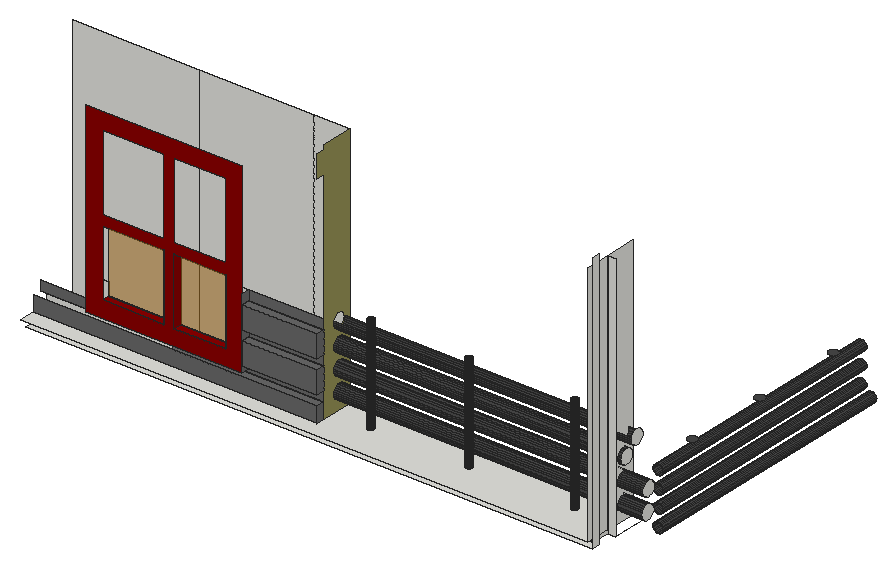
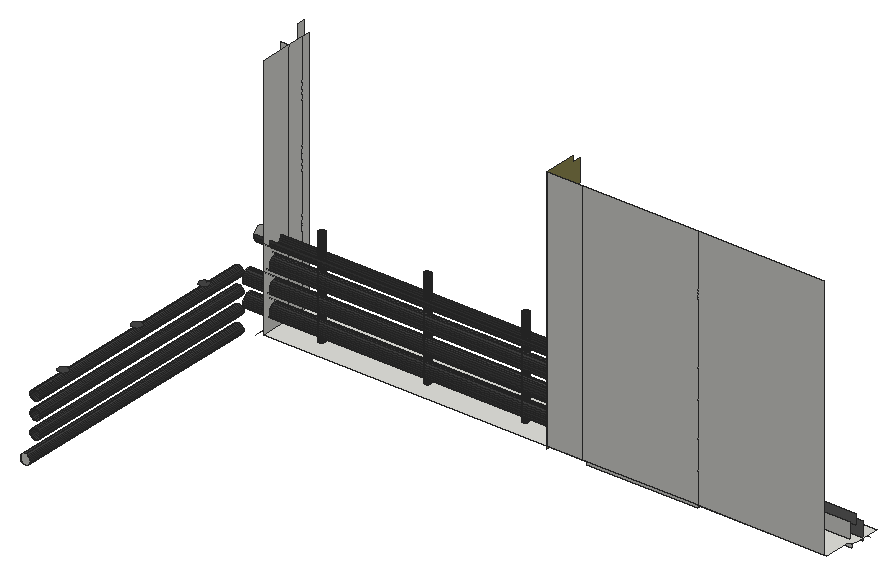
# SketchUp Ruby script. Lengths in inches.
U = 1.inch
M = Sketchup.active_model
def pt(a) = Geom::Point3d.new(a.map { |v| v * U })
def face(e, loops, mat)
  f = e.add_face(loops[0].map { |a| pt(a) })
  loops[1..].each { |l| e.add_face(l.map { |a| pt(a) }).erase! }
  f.material = f.back_material = mat if mat
  f
end
# faces: each face lists its corners as indices into pts; further lists are holes
def faces(e, pts, list, mat = nil) = list.each { |f| face(e, (f[0].is_a?(Array) ? f : [f]).map { |l| l.map { |i| pts[i] } }, mat) }
# xy, xz, yz: faces in a plane at the given z, y or x. An outline is a flat list of corners, or four numbers for a rectangle; further outlines are holes
def ring(l) = l.size == 4 ? [[l[0], l[1]], [l[2], l[1]], [l[2], l[3]], [l[0], l[3]]] : l.each_slice(2).to_a
def flat(e, list, mat, &to3) = list.each { |f| face(e, (f[0].is_a?(Array) ? f : [f]).map { |l| ring(l).map { |u, v| to3.(u, v) } }, mat) }
def xy(e, z, list, mat = nil) = flat(e, list, mat) { |x, y| [x, y, z] }
def xz(e, y, list, mat = nil) = flat(e, list, mat) { |x, z| [x, y, z] }
def yz(e, x, list, mat = nil) = flat(e, list, mat) { |y, z| [x, y, z] }
def lines(e, pts, list) = list.each { |a, b| e.add_line(pt(pts[a]), pt(pts[b])) }
# prism: a flat outline (further loops are holes) pulled along v
def prism(e, loops, v, mat = nil)
  f = face(e, loops, mat); d = Geom::Vector3d.new(v.map { |x| x * U })
  f.pushpull(f.normal.samedirection?(d) ? d.length : -d.length)
end
def box(e, o, s, mat = nil) = prism(e, [[o, [o[0] + s[0], o[1], o[2]], [o[0] + s[0], o[1] + s[1], o[2]], [o[0], o[1] + s[1], o[2]]]], [0, 0, s[2]], mat)
def at(x, y, z, deg = 0) = Geom::Transformation.translation(pt([x, y, z])) * Geom::Transformation.rotation(ORIGIN, Z_AXIS, deg.degrees)
def axes(o, x, y, z) = Geom::Transformation.new([*x, 0, *y, 0, *z, 0, *pt(o).to_a, 1])
def part(name) = M.definitions.add(name)
# library, detail: a bought-in or finely detailed component or shape, given as its bounding box
def library(name, o, s) = part(name).tap { |d| box(d.entities, o, s) }
def detail(e, o, s) = box(e.add_group.entities, o, s)
def put(e, d, t, mat = nil) = e.add_instance(d, t).tap { |i| i.material = mat if mat }
def group(e, t, mat = nil) = e.add_group.tap { |g| g.transformation = t; g.material = mat if mat }.entities
root = M.entities
M.materials.add("[0021_DarkRed]").color = [139, 0, 0]
M.materials.add("[0057_DarkKhaki]").color = [150, 145, 85]
M.materials.add("[0134_DimGray]").color = [105, 105, 105]
M.materials.add("[0137_Black]").color = [71, 71, 71]
M.materials.add("[Translucent Glass Gray]").color = [191, 123, 24]
M.materials["[Translucent Glass Gray]"].alpha = 0.5
xy(root,135.48,[[286.64,1.0625,497.29,4.0625]])
xy(root,135.98,[[286.99,7.0625,334.1,10.0625],[334.1,7.0625,375.29,10.0625],[375.29,7.0625,390.0625,10.0625],[334.1,10.0625,375.29,22.0625]])
xy(root,137.03,[[[284.41,1.0625,495.71,1.0625,495.71,22.0625,286.17,22.0625,286.17,12.1875,284.66,12.1875,284.66,10.0625,284.41,10.0625],[480.14,13.19,479.85,13.23,479.58,13.34,479.35,13.52,479.17,13.76,479.05,14.03,479.02,14.32,479.05,14.61,479.17,14.88,479.35,15.11,479.58,15.29,479.85,15.41,480.14,15.44,480.43,15.41,480.7,15.29,480.9375,15.11,481.12,14.88,481.23,14.61,481.27,14.32,481.23,14.03,481.12,13.76,480.9375,13.52,480.7,13.34,480.43,13.23],[440.77,13.19,440.47,13.23,440.2,13.34,439.97,13.52,439.79,13.76,439.68,14.03,439.64,14.32,439.68,14.61,439.79,14.88,439.97,15.11,440.2,15.29,440.47,15.41,440.77,15.44,441.06,15.41,441.33,15.29,441.5625,15.11,441.74,14.88,441.85,14.61,441.89,14.32,441.85,14.03,441.74,13.76,441.5625,13.52,441.33,13.34,441.06,13.23],[404.27,13.19,403.97,13.23,403.7,13.34,403.47,13.52,403.29,13.76,403.18,14.03,403.14,14.32,403.18,14.61,403.29,14.88,403.47,15.11,403.7,15.29,403.97,15.41,404.27,15.44,404.56,15.41,404.83,15.29,405.0625,15.11,405.24,14.88,405.35,14.61,405.39,14.32,405.35,14.03,405.24,13.76,405.0625,13.52,404.83,13.34,404.56,13.23]]])
xy(root,142.6875,[[335.53,7.0625,390.0625,10.0625]],"[0134_DimGray]")
xy(root,143.85,[[304.13,7.0625,362.13,10.0625]])
xy(root,146.27,[[362.13,7.0625,390.0625,10.0625]],"[0134_DimGray]")
xy(root,149.85,[[310.13,7.0625,333.13,10.0625],[336.9,7.0625,356.13,10.0625]],"[0021_DarkRed]")
xy(root,154.6875,[[362.13,7.0625,390.0625,10.0625]],"[0134_DimGray]")
xy(root,158.25,[[504.72,36.55,505.18,36.6,505.6,36.78,505.96,37.06,506.24,37.42,506.41,37.84,506.47,38.3,506.41,38.75,506.24,39.17,505.96,39.53,505.6,39.8125,505.18,39.99,504.72,40.05,504.27,39.99,503.85,39.8125,503.49,39.53,503.21,39.17,503.03,38.75,502.97,38.3,503.03,37.84,503.21,37.42,503.49,37.06,503.85,36.78,504.27,36.6],[504.72,67.92,505.18,67.98,505.6,68.15,505.96,68.43,506.24,68.8,506.41,69.22,506.47,69.67,506.41,70.125,506.24,70.55,505.96,70.91,505.6,71.1875,505.18,71.36,504.72,71.42,504.27,71.36,503.85,71.1875,503.49,70.91,503.21,70.55,503.03,70.125,502.97,69.67,503.03,69.22,503.21,68.8,503.49,68.43,503.85,68.15,504.27,67.98],[504.72,102.17,505.18,102.23,505.6,102.4,505.96,102.68,506.24,103.05,506.41,103.47,506.47,103.92,506.41,104.375,506.24,104.8,505.96,105.16,505.6,105.4375,505.18,105.61,504.72,105.67,504.27,105.61,503.85,105.4375,503.49,105.16,503.21,104.8,503.03,104.375,502.97,103.92,503.03,103.47,503.21,103.05,503.49,102.68,503.85,102.4,504.27,102.23]],"[0137_Black]")
xy(root,158.27,[[362.13,7.0625,390.0625,10.0625]],"[0134_DimGray]")
xy(root,166.6875,[[362.13,7.0625,390.0625,10.0625]],"[0134_DimGray]")
xz(root,7.0625,[[[304.13,143.85,362.13,212.79],[310.13,178.32,333.13,206.79],[310.13,149.85,333.13,174.59],[336.9,178.32,356.13,206.79],[336.9,149.85,356.13,174.59]]],"[0021_DarkRed]")
xz(root,7.0625,[[284.66,135.98,390.0625,142.6875],[362.13,146.27,390.0625,154.6875],[362.13,158.27,390.0625,166.6875]],"[0134_DimGray]")
xz(root,10.0625,[[286.17,134.27,390.0625,135.98],[286.99,135.98,390.0625,142.6875],[495.71,135.98,498.65,228.47],[304.13,143.85,362.13,146.27],[304.13,146.27,362.13,146.27,362.13,154.6875,356.13,154.6875,356.13,149.85,336.9,149.85,336.9,154.6875,333.13,154.6875,333.13,149.85,310.13,149.85,310.13,154.6875,304.13,154.6875],
  [362.13,146.27,390.0625,154.6875],[333.13,154.6875,336.9,158.27],[356.13,154.6875,362.13,158.27],[333.13,158.27,336.9,166.6875],[356.13,158.27,362.13,166.6875],
  [362.13,158.27,390.0625,166.6875],[333.13,166.6875,336.9,170.27],[356.13,166.6875,362.13,170.27]])
xz(root,10.0625,[[284.66,142.6875,390.0625,142.6875,390.0625,146.27,362.13,146.27,362.13,143.85,304.13,143.85,304.13,146.27,284.66,146.27],[362.13,154.6875,390.0625,158.27],[362.13,166.6875,390.0625,170.27]],"[0134_DimGray]")
xz(root,10.0625,[[310.13,149.85,333.13,174.59],[336.9,149.85,356.13,174.59]],"[Translucent Glass Gray]")
xz(root,22.0625,[[334.1,135.98,375.29,137.03],[286.99,137.03,334.1,228.47],[334.1,137.03,376.99,228.47],[376.99,137.03,390.0625,228.47]])
xz(root,121.25,[[504.95,134,504.46,134.0625,504.01,134.25,503.62,134.55,503.32,134.9375,503.14,135.39,503.07,135.875,503.14,136.36,503.32,136.8125,503.62,137.2,504.01,137.5,504.46,137.69,504.95,137.75,505.43,137.69,505.88,137.5,506.27,137.2,506.57,136.8125,506.76,136.36,506.82,135.875,506.76,135.39,506.57,134.9375,506.27,134.55,505.88,134.25,505.43,134.0625]])
yz(root,333.13,[[7.0625,149.85,10.0625,174.59]],"[0021_DarkRed]")
yz(root,336.9,[[7.0625,149.85,10.0625,174.59]],"[0021_DarkRed]")
yz(root,356.13,[[7.0625,149.85,10.0625,174.59]],"[0021_DarkRed]")
yz(root,362.13,[[7.0625,146.27,10.0625,154.6875],[7.0625,158.27,10.0625,166.6875]])
yz(root,362.13,[[7.0625,143.85,10.0625,146.27],[7.0625,154.6875,10.0625,158.27],[7.0625,166.6875,10.0625,170.27]],"[0134_DimGray]")
yz(root,390.0625,[[[10.0625,135.98,22.0625,135.98,22.0625,228.47,10.0625,228.47,10.0625,226.6875,7.0625,226.6875,7.0625,218.27,10.0625,218.27],[17.12,140.72,16.4375,140.81,15.81,141.07,15.26,141.49,14.85,142.03,14.58,142.66,14.49,143.34,14.58,144.02,14.85,144.66,15.26,145.2,15.81,145.62,16.4375,145.88,17.12,145.97,17.8,145.88,18.43,145.62,18.97,145.2,19.39,144.66,19.65,144.02,19.74,143.34,19.65,142.66,19.39,142.03,18.97,141.49,18.43,141.07,17.8,140.81],[17.12,148.59,16.4375,148.68,15.81,148.95,15.26,149.36,14.85,149.91,14.58,150.54,14.49,151.22,14.58,151.9,14.85,152.53,15.26,153.08,15.81,153.49,16.4375,153.75,17.12,153.84,17.8,153.75,18.43,153.49,18.97,153.08,19.39,152.53,19.65,151.9,19.74,151.22,19.65,150.54,19.39,149.91,18.97,149.36,18.43,148.95,17.8,148.68],[17.12,156.47,16.4375,156.56,15.81,156.82,15.26,157.24,14.85,157.78,14.58,158.41,14.49,159.09,14.58,159.77,14.85,160.41,15.26,160.95,15.81,161.37,16.4375,161.63,17.12,161.72,17.8,161.63,18.43,161.37,18.97,160.95,19.39,160.41,19.65,159.77,19.74,159.09,19.65,158.41,19.39,157.78,18.97,157.24,18.43,156.82,17.8,156.56],[17.12,164.34,16.4375,164.43,15.81,164.7,15.26,165.11,14.85,165.66,14.58,166.29,14.49,166.97,14.58,167.65,14.85,168.28,15.26,168.83,15.81,169.24,16.4375,169.5,17.12,169.59,17.8,169.5,18.43,169.24,18.97,168.83,19.39,168.28,19.65,167.65,19.74,166.97,19.65,166.29,19.39,165.66,18.97,165.11,18.43,164.7,17.8,164.43]]],"[0057_DarkKhaki]")
yz(root,390.0625,[[7.0625,135.98,10.0625,142.6875],[7.0625,146.27,10.0625,154.6875],[7.0625,158.27,10.0625,166.6875]],"[0134_DimGray]")
yz(root,495.71,[[4.0625,135.98,10.0625,137.03],[1.0625,137.03,4.0625,228.47],[4.0625,137.03,10.0625,228.47],[10.0625,137.03,22.0625,228.47]])
yz(root,497.29,[[1.0625,135.48,4.0625,232.22],[17.12,156.47,17.8,156.56,18.43,156.82,18.97,157.24,19.39,157.78,19.65,158.41,19.74,159.09,19.65,159.77,19.39,160.41,18.97,160.95,18.43,161.37,17.8,161.63,17.12,161.72,16.4375,161.63,15.81,161.37,15.26,160.95,14.85,160.41,14.58,159.77,14.49,159.09,14.58,158.41,14.85,157.78,15.26,157.24,15.81,156.82,16.4375,156.56]])
yz(root,501.0625,[[17.12,164.34,17.8,164.43,18.43,164.7,18.97,165.11,19.39,165.66,19.65,166.29,19.74,166.97,19.65,167.65,19.39,168.28,18.97,168.83,18.43,169.24,17.8,169.5,17.12,169.59,16.4375,169.5,15.81,169.24,15.26,168.83,14.85,168.28,14.58,167.65,14.49,166.97,14.58,166.29,14.85,165.66,15.26,165.11,15.81,164.7,16.4375,164.43]])
yz(root,505.125,[[17.12,140.72,17.8,140.81,18.43,141.07,18.97,141.49,19.39,142.03,19.65,142.66,19.74,143.34,19.65,144.02,19.39,144.66,18.97,145.2,18.43,145.62,17.8,145.88,17.12,145.97,16.4375,145.88,15.81,145.62,15.26,145.2,14.85,144.66,14.58,144.02,14.49,143.34,14.58,142.66,14.85,142.03,15.26,141.49,15.81,141.07,16.4375,140.81]])
yz(root,505.375,[[17.12,148.59,17.8,148.68,18.43,148.95,18.97,149.36,19.39,149.91,19.65,150.54,19.74,151.22,19.65,151.9,19.39,152.53,18.97,153.08,18.43,153.49,17.8,153.75,17.12,153.84,16.4375,153.75,15.81,153.49,15.26,153.08,14.85,152.53,14.58,151.9,14.49,151.22,14.58,150.54,14.85,149.91,15.26,149.36,15.81,148.95,16.4375,148.68]])
p = [[504.95,22.0625,134],[504.46,22.0625,134.0625],[504.46,121.25,134.0625],[504.95,121.25,134],[505.43,22.0625,134.0625],[505.43,121.25,134.0625],
  [504.01,22.0625,134.25],[504.01,121.25,134.25],[505.88,22.0625,134.25],[505.88,121.25,134.25],[503.62,22.0625,134.55],[503.62,121.25,134.55],
  [506.27,22.0625,134.55],[506.27,121.25,134.55],[503.32,22.0625,134.9375],[503.32,121.25,134.9375],[506.57,22.0625,134.9375],[506.57,121.25,134.9375],
  [503.14,22.0625,135.39],[503.14,121.25,135.39],[506.76,22.0625,135.39],[506.76,121.25,135.39],[503.07,22.0625,135.875],[503.07,121.25,135.875],
  [506.82,22.0625,135.875],[506.82,121.25,135.875],[503.14,22.0625,136.36],[503.14,121.25,136.36],[506.76,22.0625,136.36],[506.76,121.25,136.36],
  [503.32,22.0625,136.8125],[503.32,121.25,136.8125],[506.57,22.0625,136.8125],[506.57,121.25,136.8125],[503.62,22.0625,137.2],[503.62,121.25,137.2],
  [506.27,22.0625,137.2],[506.27,121.25,137.2],[403.7,13.34,137.03],[403.97,13.23,137.03],[403.97,13.23,173.53],[403.7,13.34,173.53],
  [404.27,13.19,137.03],[404.27,13.19,173.53],[404.56,13.23,137.03],[404.56,13.23,173.53],[404.83,13.34,137.03],[404.83,13.34,173.53],
  [440.2,13.34,137.03],[440.47,13.23,137.03],[440.47,13.23,173.53],[440.2,13.34,173.53],[440.77,13.19,137.03],[440.77,13.19,173.53],
  [441.06,13.23,137.03],[441.06,13.23,173.53],[441.33,13.34,137.03],[441.33,13.34,173.53],[479.58,13.34,137.03],[479.85,13.23,137.03],
  [479.85,13.23,173.53],[479.58,13.34,173.53],[480.14,13.19,137.03],[480.14,13.19,173.53],[480.43,13.23,137.03],[480.43,13.23,173.53],
  [480.7,13.34,137.03],[480.7,13.34,173.53],[403.47,13.52,137.03],[403.47,13.52,173.53],[405.0625,13.52,137.03],[405.0625,13.52,173.53],
  [439.97,13.52,137.03],[439.97,13.52,173.53],[441.5625,13.52,137.03],[441.5625,13.52,173.53],[479.35,13.52,137.03],[479.35,13.52,173.53],
  [480.9375,13.52,137.03],[480.9375,13.52,173.53],[403.29,13.76,137.03],[403.29,13.76,173.53],[405.24,13.76,137.03],[405.24,13.76,173.53],
  [439.79,13.76,137.03],[439.79,13.76,173.53],[441.74,13.76,137.03],[441.74,13.76,173.53],[479.17,13.76,137.03],[479.17,13.76,173.53],
  [481.12,13.76,137.03],[481.12,13.76,173.53],[403.18,14.03,137.03],[403.18,14.03,173.53],[405.35,14.03,137.03],[405.35,14.03,173.53],
  [439.68,14.03,137.03],[439.68,14.03,173.53],[441.85,14.03,137.03],[441.85,14.03,173.53],[479.05,14.03,137.03],[479.05,14.03,173.53],
  [481.23,14.03,137.03],[481.23,14.03,173.53],[403.14,14.32,137.03],[403.14,14.32,173.53],[405.39,14.32,137.03],[405.39,14.32,173.53],
  [439.64,14.32,137.03],[439.64,14.32,173.53],[441.89,14.32,137.03],[441.89,14.32,173.53],[479.02,14.32,137.03],[479.02,14.32,173.53],
  [481.27,14.32,137.03],[481.27,14.32,173.53],[403.18,14.61,137.03],[403.18,14.61,173.53],[405.35,14.61,137.03],[405.35,14.61,173.53],
  [439.68,14.61,137.03],[439.68,14.61,173.53],[441.85,14.61,137.03],[441.85,14.61,173.53],[479.05,14.61,137.03],[479.05,14.61,173.53],
  [481.23,14.61,137.03],[481.23,14.61,173.53],[403.29,14.88,137.03],[403.29,14.88,173.53],[405.24,14.88,137.03],[405.24,14.88,173.53],
  [439.79,14.88,137.03],[439.79,14.88,173.53],[441.74,14.88,137.03],[441.74,14.88,173.53],[479.17,14.88,137.03],[479.17,14.88,173.53],
  [481.12,14.88,137.03],[481.12,14.88,173.53],[403.47,15.11,137.03],[403.47,15.11,173.53],[405.0625,15.11,137.03],[405.0625,15.11,173.53],
  [439.97,15.11,137.03],[439.97,15.11,173.53],[441.5625,15.11,137.03],[441.5625,15.11,173.53],[479.35,15.11,137.03],[479.35,15.11,173.53],
  [480.9375,15.11,137.03],[480.9375,15.11,173.53],[403.7,15.29,137.03],[403.7,15.29,173.53],[404.83,15.29,137.03],[404.83,15.29,173.53],
  [440.2,15.29,137.03],[440.2,15.29,173.53],[441.33,15.29,137.03],[441.33,15.29,173.53],[479.58,15.29,137.03],[479.58,15.29,173.53],
  [480.7,15.29,137.03],[480.7,15.29,173.53],[403.97,15.41,137.03],[403.97,15.41,173.53],[404.56,15.41,137.03],[404.56,15.41,173.53],
  [440.47,15.41,137.03],[440.47,15.41,173.53],[441.06,15.41,137.03],[441.06,15.41,173.53],[479.85,15.41,137.03],[479.85,15.41,173.53],
  [480.43,15.41,137.03],[480.43,15.41,173.53],[404.27,15.44,137.03],[404.27,15.44,173.53],[440.77,15.44,137.03],[440.77,15.44,173.53],
  [480.14,15.44,137.03],[480.14,15.44,173.53],[504.01,22.0625,137.5],[504.01,121.25,137.5],[505.88,22.0625,137.5],[505.88,121.25,137.5],
  [504.46,22.0625,137.69],[504.46,121.25,137.69],[505.43,22.0625,137.69],[505.43,121.25,137.69],[504.95,22.0625,137.75],[504.95,121.25,137.75],
  [504.95,22.0625,140.4375],[504.46,22.0625,140.5],[504.46,116.75,140.5],[504.95,116.75,140.4375],[505.43,22.0625,140.5],[505.43,116.75,140.5],
  [504.01,22.0625,140.6875],[504.01,116.75,140.6875],[505.88,22.0625,140.6875],[505.88,116.75,140.6875],[390.0625,16.4375,140.81],[390.0625,17.12,140.72],
  [505.125,17.12,140.72],[505.125,16.4375,140.81],[390.0625,17.8,140.81],[505.125,17.8,140.81],[503.62,22.0625,140.99],[503.62,116.75,140.99],
  [506.27,22.0625,140.99],[506.27,116.75,140.99],[390.0625,15.81,141.07],[505.125,15.81,141.07],[390.0625,18.43,141.07],[505.125,18.43,141.07],
  [503.32,22.0625,141.375],[503.32,116.75,141.375],[506.57,22.0625,141.375],[506.57,116.75,141.375],[390.0625,15.26,141.49],[505.125,15.26,141.49],
  [390.0625,18.97,141.49],[505.125,18.97,141.49],[503.14,22.0625,141.83],[503.14,116.75,141.83],[506.76,22.0625,141.83],[506.76,116.75,141.83],
  [390.0625,14.85,142.03],[505.125,14.85,142.03],[390.0625,19.39,142.03],[505.125,19.39,142.03],[503.07,22.0625,142.3125],[503.07,116.75,142.3125],
  [506.82,22.0625,142.3125],[506.82,116.75,142.3125],[390.0625,14.58,142.66],[505.125,14.58,142.66],[390.0625,19.65,142.66],[505.125,19.65,142.66],
  [503.14,22.0625,142.8],[503.14,116.75,142.8],[506.76,22.0625,142.8],[506.76,116.75,142.8],[390.0625,14.49,143.34],[505.125,14.49,143.34],
  [390.0625,19.74,143.34],[505.125,19.74,143.34],[503.32,22.0625,143.25],[503.32,116.75,143.25],[506.57,22.0625,143.25],[506.57,116.75,143.25],
  [503.62,22.0625,143.64],[503.62,116.75,143.64],[506.27,22.0625,143.64],[506.27,116.75,143.64],[390.0625,14.58,144.02],[505.125,14.58,144.02],
  [390.0625,19.65,144.02],[505.125,19.65,144.02],[504.01,22.0625,143.9375],[504.01,116.75,143.9375],[505.88,22.0625,143.9375],[505.88,116.75,143.9375],
  [504.46,22.0625,144.12],[504.46,116.75,144.12],[505.43,22.0625,144.12],[505.43,116.75,144.12],[390.0625,14.85,144.66],[505.125,14.85,144.66],
  [390.0625,19.39,144.66],[505.125,19.39,144.66],[504.95,22.0625,144.1875],[504.95,116.75,144.1875],[390.0625,15.26,145.2],[505.125,15.26,145.2],
  [390.0625,18.97,145.2],[505.125,18.97,145.2],[390.0625,15.81,145.62],[505.125,15.81,145.62],[390.0625,18.43,145.62],[505.125,18.43,145.62],
  [390.0625,16.4375,145.88],[505.125,16.4375,145.88],[390.0625,17.8,145.88],[505.125,17.8,145.88],[390.0625,17.12,145.97],[505.125,17.12,145.97],
  [504.46,22.0625,146.9375],[504.01,22.0625,147.125],[504.01,116.75,147.125],[504.46,116.75,146.9375],[504.95,22.0625,146.875],[504.95,116.75,146.875],
  [505.43,22.0625,146.9375],[505.43,116.75,146.9375],[505.88,22.0625,147.125],[505.88,116.75,147.125],[503.62,22.0625,147.42],[503.62,116.75,147.42],
  [506.27,22.0625,147.42],[506.27,116.75,147.42],[503.32,22.0625,147.8125],[503.32,116.75,147.8125],[506.57,22.0625,147.8125],[506.57,116.75,147.8125],
  [503.14,22.0625,148.26],[503.14,116.75,148.26],[506.76,22.0625,148.26],[506.76,116.75,148.26],[503.07,22.0625,148.75],[503.07,116.75,148.75],
  [506.82,22.0625,148.75],[506.82,116.75,148.75],[390.0625,16.4375,148.68],[390.0625,17.12,148.59],[505.375,17.12,148.59],[505.375,16.4375,148.68],
  [390.0625,17.8,148.68],[505.375,17.8,148.68],[390.0625,15.81,148.95],[505.375,15.81,148.95],[390.0625,18.43,148.95],[505.375,18.43,148.95],
  [503.14,22.0625,149.23],[503.14,116.75,149.23],[506.76,22.0625,149.23],[506.76,116.75,149.23],[390.0625,15.26,149.36],[505.375,15.26,149.36],
  [390.0625,18.97,149.36],[505.375,18.97,149.36],[503.32,22.0625,149.6875],[503.32,116.75,149.6875],[506.57,22.0625,149.6875],[506.57,116.75,149.6875],
  [390.0625,14.85,149.91],[505.375,14.85,149.91],[390.0625,19.39,149.91],[505.375,19.39,149.91],[503.62,22.0625,150.08],[503.62,116.75,150.08],
  [506.27,22.0625,150.08],[506.27,116.75,150.08],[390.0625,14.58,150.54],[505.375,14.58,150.54],[390.0625,19.65,150.54],[505.375,19.65,150.54],
  [504.01,22.0625,150.375],[504.01,116.75,150.375],[505.88,22.0625,150.375],[505.88,116.75,150.375],[504.46,22.0625,150.56],[504.46,116.75,150.56],
  [505.43,22.0625,150.56],[505.43,116.75,150.56],[390.0625,14.49,151.22],[505.375,14.49,151.22],[390.0625,19.74,151.22],[505.375,19.74,151.22],
  [504.95,22.0625,150.625],[504.95,116.75,150.625],[390.0625,14.58,151.9],[505.375,14.58,151.9],[390.0625,19.65,151.9],[505.375,19.65,151.9],
  [390.0625,14.85,152.53],[505.375,14.85,152.53],[390.0625,19.39,152.53],[505.375,19.39,152.53],[390.0625,15.26,153.08],[505.375,15.26,153.08],
  [390.0625,18.97,153.08],[505.375,18.97,153.08],[390.0625,15.81,153.49],[505.375,15.81,153.49],[390.0625,18.43,153.49],[505.375,18.43,153.49],
  [504.95,22.0625,153.3125],[504.46,22.0625,153.375],[504.46,116.75,153.375],[504.95,116.75,153.3125],[505.43,22.0625,153.375],[505.43,116.75,153.375],
  [504.01,22.0625,153.5625],[504.01,116.75,153.5625],[505.88,22.0625,153.5625],[505.88,116.75,153.5625],[390.0625,16.4375,153.75],[505.375,16.4375,153.75],
  [390.0625,17.8,153.75],[505.375,17.8,153.75],[503.62,22.0625,153.86],[503.62,116.75,153.86],[506.27,22.0625,153.86],[506.27,116.75,153.86],
  [390.0625,17.12,153.84],[505.375,17.12,153.84],[503.32,22.0625,154.25],[503.32,116.75,154.25],[506.57,22.0625,154.25],[506.57,116.75,154.25],
  [503.14,22.0625,154.7],[503.14,116.75,154.7],[506.76,22.0625,154.7],[506.76,116.75,154.7],[503.07,22.0625,155.1875],[503.07,116.75,155.1875],
  [506.82,22.0625,155.1875],[506.82,116.75,155.1875],[503.14,22.0625,155.67],[503.14,116.75,155.67],[506.76,22.0625,155.67],[506.76,116.75,155.67],
  [503.32,22.0625,156.125],[503.32,116.75,156.125],[506.57,22.0625,156.125],[506.57,116.75,156.125],[503.62,22.0625,156.51],[503.62,116.75,156.51],
  [506.27,22.0625,156.51],[506.27,116.75,156.51],[390.0625,16.4375,156.56],[390.0625,17.12,156.47],[497.29,17.12,156.47],[497.29,16.4375,156.56],
  [390.0625,17.8,156.56],[497.29,17.8,156.56],[504.01,22.0625,156.8125],[504.01,116.75,156.8125],[505.88,22.0625,156.8125],[505.88,116.75,156.8125],
  [390.0625,15.81,156.82],[497.29,15.81,156.82],[390.0625,18.43,156.82],[497.29,18.43,156.82],[390.0625,15.26,157.24],[497.29,15.26,157.24],
  [390.0625,18.97,157.24],[497.29,18.97,157.24],[504.46,22.0625,157],[504.46,116.75,157],[505.43,22.0625,157],[505.43,116.75,157],
  [504.95,22.0625,157.0625],[504.95,116.75,157.0625],[390.0625,14.85,157.78],[497.29,14.85,157.78],[390.0625,19.39,157.78],[497.29,19.39,157.78],
  [390.0625,14.58,158.41],[497.29,14.58,158.41],[390.0625,19.65,158.41],[497.29,19.65,158.41],[390.0625,14.49,159.09],[497.29,14.49,159.09],
  [390.0625,19.74,159.09],[497.29,19.74,159.09],[390.0625,14.58,159.77],[497.29,14.58,159.77],[390.0625,19.65,159.77],[497.29,19.65,159.77],
  [390.0625,14.85,160.41],[497.29,14.85,160.41],[390.0625,19.39,160.41],[497.29,19.39,160.41],[390.0625,15.26,160.95],[497.29,15.26,160.95],
  [390.0625,18.97,160.95],[497.29,18.97,160.95],[390.0625,15.81,161.37],[497.29,15.81,161.37],[390.0625,18.43,161.37],[497.29,18.43,161.37],
  [390.0625,16.4375,161.63],[497.29,16.4375,161.63],[390.0625,17.8,161.63],[497.29,17.8,161.63],[390.0625,17.12,161.72],[497.29,17.12,161.72],
  [390.0625,16.4375,164.43],[390.0625,17.12,164.34],[501.0625,17.12,164.34],[501.0625,16.4375,164.43],[390.0625,17.8,164.43],[501.0625,17.8,164.43],
  [390.0625,15.81,164.7],[501.0625,15.81,164.7],[390.0625,18.43,164.7],[501.0625,18.43,164.7],[390.0625,15.26,165.11],[501.0625,15.26,165.11],
  [390.0625,18.97,165.11],[501.0625,18.97,165.11],[390.0625,14.85,165.66],[501.0625,14.85,165.66],[390.0625,19.39,165.66],[501.0625,19.39,165.66],
  [390.0625,14.58,166.29],[501.0625,14.58,166.29],[390.0625,19.65,166.29],[501.0625,19.65,166.29],[390.0625,14.49,166.97],[501.0625,14.49,166.97],
  [390.0625,19.74,166.97],[501.0625,19.74,166.97],[390.0625,14.58,167.65],[501.0625,14.58,167.65],[390.0625,19.65,167.65],[501.0625,19.65,167.65],
  [495.71,4.0625,135.98],[284.41,4.0625,135.98],[498.65,22.0625,135.98],[498.65,10.0625,135.98]]
faces(root,p,[[0,1,2,3],[4,0,3,5],[1,6,7,2],[8,4,5,9],[6,10,11,7],[12,8,9,13],[10,14,15,11],[16,12,13,17],
  [14,18,19,15],[20,16,17,21],[18,22,23,19],[24,20,21,25],[22,26,27,23],[28,24,25,29],[26,30,31,27],[32,28,29,33],
  [30,34,35,31],[36,32,33,37],[38,39,40,41],[39,42,43,40],[42,44,45,43],[44,46,47,45],[48,49,50,51],[49,52,53,50],
  [52,54,55,53],[54,56,57,55],[58,59,60,61],[59,62,63,60],[62,64,65,63],[64,66,67,65],[68,38,41,69],[46,70,71,47],
  [72,48,51,73],[56,74,75,57],[76,58,61,77],[66,78,79,67],[80,68,69,81],[70,82,83,71],[84,72,73,85],[74,86,87,75],
  [88,76,77,89],[78,90,91,79],[92,80,81,93],[82,94,95,83],[96,84,85,97],[86,98,99,87],[100,88,89,101],[90,102,103,91],
  [104,92,93,105],[94,106,107,95],[108,96,97,109],[98,110,111,99],[112,100,101,113],[102,114,115,103],[116,104,105,117],[106,118,119,107],
  [120,108,109,121],[110,122,123,111],[124,112,113,125],[114,126,127,115],[128,116,117,129],[118,130,131,119],[132,120,121,133],[122,134,135,123],
  [136,124,125,137],[126,138,139,127],[140,128,129,141],[130,142,143,131],[144,132,133,145],[134,146,147,135],[148,136,137,149],[138,150,151,139],
  [152,140,141,153],[142,154,155,143],[156,144,145,157],[146,158,159,147],[160,148,149,161],[150,162,163,151],[164,152,153,165],[154,166,167,155],
  [168,156,157,169],[158,170,171,159],[172,160,161,173],[162,174,175,163],[176,164,165,177],[166,176,177,167],[178,168,169,179],[170,178,179,171],
  [180,172,173,181],[174,180,181,175],[34,182,183,35],[184,36,37,185],[182,186,187,183],[188,184,185,189],[186,190,191,187],[190,188,189,191],
  [192,193,194,195],[196,192,195,197],[193,198,199,194],[200,196,197,201],[202,203,204,205],[203,206,207,204],[198,208,209,199],[210,200,201,211],
  [212,202,205,213],[206,214,215,207],[208,216,217,209],[218,210,211,219],[220,212,213,221],[214,222,223,215],[216,224,225,217],[226,218,219,227],
  [228,220,221,229],[222,230,231,223],[224,232,233,225],[234,226,227,235],[236,228,229,237],[230,238,239,231],[232,240,241,233],[242,234,235,243],
  [244,236,237,245],[238,246,247,239],[240,248,249,241],[250,242,243,251],[248,252,253,249],[254,250,251,255],[256,244,245,257],[246,258,259,247],
  [252,260,261,253],[262,254,255,263],[260,264,265,261],[266,262,263,267],[268,256,257,269],[258,270,271,259],[264,272,273,265],[272,266,267,273],
  [274,268,269,275],[270,276,277,271],[278,274,275,279],[276,280,281,277],[282,278,279,283],[280,284,285,281],[286,282,283,287],[284,286,287,285],
  [288,289,290,291],[292,288,291,293],[294,292,293,295],[296,294,295,297],[289,298,299,290],[300,296,297,301],[298,302,303,299],[304,300,301,305],
  [302,306,307,303],[308,304,305,309],[306,310,311,307],[312,308,309,313],[314,315,316,317],[315,318,319,316],[320,314,317,321],[318,322,323,319],
  [310,324,325,311],[326,312,313,327],[328,320,321,329],[322,330,331,323],[324,332,333,325],[334,326,327,335],[336,328,329,337],[330,338,339,331],
  [332,340,341,333],[342,334,335,343],[344,336,337,345],[338,346,347,339],[340,348,349,341],[350,342,343,351],[348,352,353,349],[354,350,351,355],
  [356,344,345,357],[346,358,359,347],[352,360,361,353],[360,354,355,361],[362,356,357,363],[358,364,365,359],[366,362,363,367],[364,368,369,365],
  [370,366,367,371],[368,372,373,369],[374,370,371,375],[372,376,377,373],[378,379,380,381],[382,378,381,383],[379,384,385,380],[386,382,383,387],
  [388,374,375,389],[376,390,391,377],[384,392,393,385],[394,386,387,395],[396,388,389,397],[390,396,397,391],[392,398,399,393],[400,394,395,401],
  [398,402,403,399],[404,400,401,405],[402,406,407,403],[408,404,405,409],[406,410,411,407],[412,408,409,413],[410,414,415,411],[416,412,413,417],
  [414,418,419,415],[420,416,417,421],[422,423,424,425],[423,426,427,424],[418,428,429,419],[430,420,421,431],[432,422,425,433],[426,434,435,427],
  [436,432,433,437],[434,438,439,435],[428,440,441,429],[442,430,431,443],[440,444,445,441],[444,442,443,445],[446,436,437,447],[438,448,449,439],
  [450,446,447,451],[448,452,453,449],[454,450,451,455],[452,456,457,453],[458,454,455,459],[456,460,461,457],[462,458,459,463],[460,464,465,461],
  [466,462,463,467],[464,468,469,465],[470,466,467,471],[468,472,473,469],[474,470,471,475],[472,476,477,473],[478,474,475,479],[476,478,479,477],
  [480,481,482,483],[481,484,485,482],[486,480,483,487],[484,488,489,485],[490,486,487,491],[488,492,493,489],[494,490,491,495],[492,496,497,493],
  [498,494,495,499],[496,500,501,497],[502,498,499,503],[500,504,505,501],[506,502,503,507],[504,508,509,505]],"[0137_Black]")
lines(root,p,[[510,511],[512,513]])
